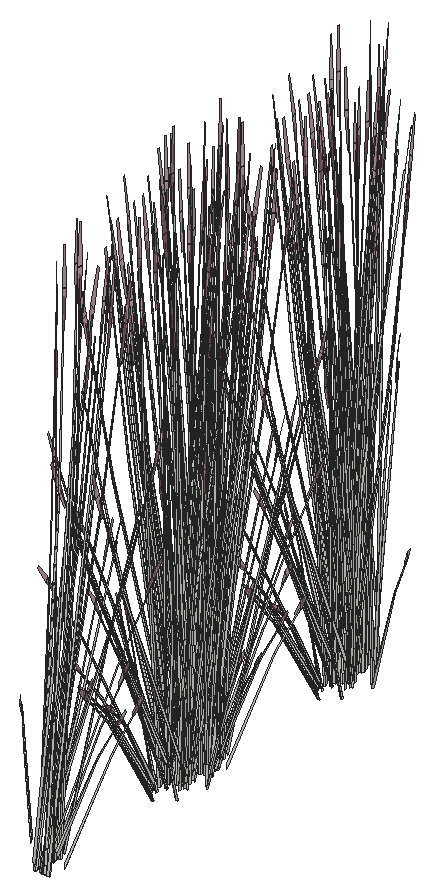
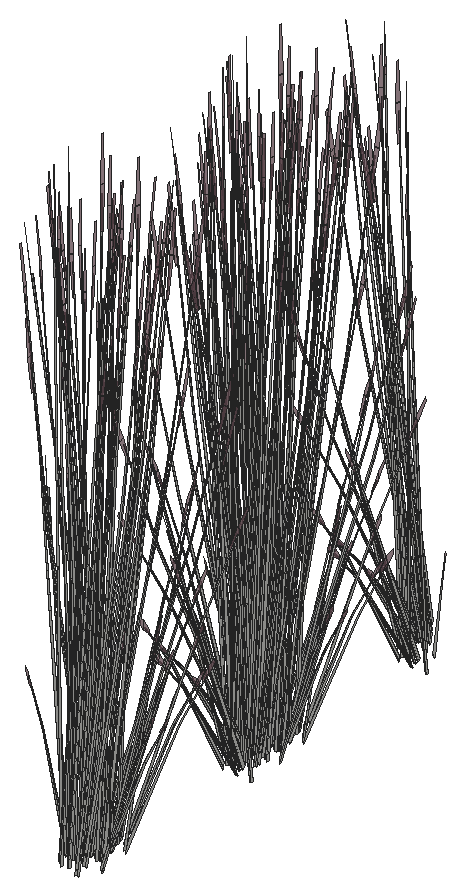
# SketchUp Ruby script. Lengths in inches.
U = 1.inch
M = Sketchup.active_model
def pt(a) = Geom::Point3d.new(a.map { |v| v * U })
def face(e, loops, mat)
  f = e.add_face(loops[0].map { |a| pt(a) })
  loops[1..].each { |l| e.add_face(l.map { |a| pt(a) }).erase! }
  f.material = f.back_material = mat if mat
  f
end
# faces: each face lists its corners as indices into pts; further lists are holes
def faces(e, pts, list, mat = nil) = list.each { |f| face(e, (f[0].is_a?(Array) ? f : [f]).map { |l| l.map { |i| pts[i] } }, mat) }
# xy, xz, yz: faces in a plane at the given z, y or x. An outline is a flat list of corners, or four numbers for a rectangle; further outlines are holes
def ring(l) = l.size == 4 ? [[l[0], l[1]], [l[2], l[1]], [l[2], l[3]], [l[0], l[3]]] : l.each_slice(2).to_a
def flat(e, list, mat, &to3) = list.each { |f| face(e, (f[0].is_a?(Array) ? f : [f]).map { |l| ring(l).map { |u, v| to3.(u, v) } }, mat) }
def xy(e, z, list, mat = nil) = flat(e, list, mat) { |x, y| [x, y, z] }
def xz(e, y, list, mat = nil) = flat(e, list, mat) { |x, z| [x, y, z] }
def yz(e, x, list, mat = nil) = flat(e, list, mat) { |y, z| [x, y, z] }
def lines(e, pts, list) = list.each { |a, b| e.add_line(pt(pts[a]), pt(pts[b])) }
# prism: a flat outline (further loops are holes) pulled along v
def prism(e, loops, v, mat = nil)
  f = face(e, loops, mat); d = Geom::Vector3d.new(v.map { |x| x * U })
  f.pushpull(f.normal.samedirection?(d) ? d.length : -d.length)
end
def box(e, o, s, mat = nil) = prism(e, [[o, [o[0] + s[0], o[1], o[2]], [o[0] + s[0], o[1] + s[1], o[2]], [o[0], o[1] + s[1], o[2]]]], [0, 0, s[2]], mat)
def at(x, y, z, deg = 0) = Geom::Transformation.translation(pt([x, y, z])) * Geom::Transformation.rotation(ORIGIN, Z_AXIS, deg.degrees)
def axes(o, x, y, z) = Geom::Transformation.new([*x, 0, *y, 0, *z, 0, *pt(o).to_a, 1])
def part(name) = M.definitions.add(name)
# library, detail: a bought-in or finely detailed component or shape, given as its bounding box
def library(name, o, s) = part(name).tap { |d| box(d.entities, o, s) }
def detail(e, o, s) = box(e.add_group.entities, o, s)
def put(e, d, t, mat = nil) = e.add_instance(d, t).tap { |i| i.material = mat if mat }
def group(e, t, mat = nil) = e.add_group.tap { |g| g.transformation = t; g.material = mat if mat }.entities
root = M.entities
M.materials.add("LightPink_Translucent").color = [144, 107, 117]
M.materials["LightPink_Translucent"].alpha = 0.75
c1 = part("blade")
p = [[2.15,0.21,22],[0,0.17,0],[0.09,0.45,0],[2.18,0.31,22],[2.29,0.31,22],[0.38,0.45,0],
  [2.48,0.24,33],[2.49,0.24,33],[2.48,0.22,33]]
faces(c1.entities,p,[[0,1,2,3],[4,5,2,3],[6,3,4,7],[8,0,3,6]])
c2 = part("seeds")
p = [[0.3,-0.1,1.38],[-0.01,-0.03,1.59],[-0.01,-0.03,0.03],[0.14,-0.07,-0.07],[0.29,-0.03,3],[0.15,0.01,3.11]]
faces(c2.entities,p,[[0,1,2,3],[1,0,4,5]],"LightPink_Translucent")
c3 = part("blade with seeds")
put(c3.entities,c1,at(0,0,0))
put(c3.entities,c2,axes([2.4,0.25,30.99],[1.5799,-0.05474,1.17369],[-0.12525,1.92788,0.29478],[-0.07173,-0.02425,1.56792]))
put(root,c3,axes([252.92,30.17,0.92],[0.32006,0,0],[0,0.68339,-0.37456],[0,0.15565,1.18819]))
put(root,c3,axes([252.79,30.52,0.79],[-0.3199,-0.00489,-0.03612],[0,-0.68339,0.36248],[-0.01005,0.15557,1.14929]))
put(root,c3,axes([252.1,29.93,1.13],[0.28825,0.29175,-0.21117],[-0.1388,0.61578,-0.36291],[0.00906,0.15119,1.15913]))
put(root,c3,axes([250.09,32.2,1.2],[0.10667,-0.27712,0.83364],[0.04209,0.43871,0.6125],[-0.07709,0.07855,0.18362]))
put(root,c3,axes([252.73,30.62,0.66],[-0.17867,0.3815,-0.22483],[-0.17867,-0.3815,0.22483],[0,0.12288,1.00865]))
put(root,c3,axes([251.96,30.66,1.13],[0.02983,0.6977,-0.21117],[-0.31064,0.04219,-0.36291],[-0.0547,0.09294,1.15913]))
put(root,c3,axes([252.07,30.39,0.8],[-0.12419,0.55096,-0.32471],[-0.25804,-0.26516,0.15627],[0,0.12701,1.04254]))
put(root,c3,axes([251.77,31.19,0.6875],[-0.1724,0.45959,-0.45255],[-0.21416,-0.41674,-0.11877],[-0.06908,0.11465,0.99892]))
put(root,c3,axes([252.08,31.97,0.88],[0.32044,0.19874,0.22322],[-0.08017,0.71038,-0.26485],[-0.05304,0.08891,1.19671]))
put(root,c3,axes([252.05,32.44,0.66],[-0.23955,0.30573,-0.36036],[-0.14318,-0.54821,0],[-0.05456,0.06963,1.14313]))
put(root,c3,axes([252.85,30.63,0.66],[0,0.61145,-0.36036],[-0.28637,0,0],[0,0.13926,1.14313]))
put(root,c3,axes([252.49,31.9,1.2],[-0.14411,-0.17581,0.83364],[0.18609,-0.17864,0.6125],[0.05019,0.15132,0.18362]))
put(root,c3,axes([252.27,32.35,0.91],[0.16003,0.61271,0],[-0.26773,0.34169,-0.37456],[-0.06098,0.07782,1.18819]))
put(root,c3,axes([252.53,32.56,0.28],[0.01865,-0.08828,1.27986],[0.23477,-0.25998,-0.19552],[0.07118,0.13456,0.218]))
put(root,c3,axes([252.13,29.92,1.26],[-0.00699,-0.5757,1.02533],[0.31645,0.14923,0.43413],[-0.07484,0.31502,0.96783]))
put(root,c3,axes([252.22,30.55,0.71],[0.09385,0.55983,-0.50233],[-0.27035,0.20162,-0.13184],[0.01037,0.18957,1.1088]))
put(root,c3,axes([250.37,32.48,0.28],[0.03433,0.06109,1.27986],[0.05822,0.56601,-0.19552],[-0.07609,0.1207,0.218]))
put(root,c3,axes([252.51,32.7,1.13],[-0.16414,-0.01918,0.76251],[0.10839,-0.40729,0.421],[0.06484,0.1447,0.59812]))
put(root,c3,axes([251.97,31.72,1.07],[0.00452,-0.20269,1.03788],[0.21585,-0.22641,-0.22321],[0.06663,0.2426,0.44375]))
put(root,c3,axes([250.99,33.41,1.2],[-0.00662,-0.36357,0.83364],[0.16552,0.25931,0.6125],[-0.03255,0.17329,0.18362]))
put(root,c3,axes([251.43,32.54,0.28],[0.04142,-0.03327,1.27986],[0.24917,0.18313,-0.19552],[0.00729,0.2064,0.218]))
put(root,c3,axes([250.86,32.62,1.24],[0.23252,-0.10828,0.04723],[0.05346,0.43623,-0.62638],[-0.01474,0.22082,0.56147]))
put(root,c3,axes([251.51,32.3,2.81],[0.12216,0.49718,-0.51563],[-0.25147,0.27708,0.06223],[0.02857,0.24022,0.72942]))
put(root,c3,axes([250.8,33.08,1.07],[0.08077,-0.09646,1.03788],[0.19942,0.29084,-0.22321],[-0.05936,0.25166,0.44375]))
put(root,c3,axes([252.15,43.34,1.07],[-0.07276,0.12376,1.03788],[-0.21789,-0.21662,-0.22321],[0.04039,-0.2694,0.44375]))
put(root,c3,axes([251.82,43.77,2.81],[-0.12216,-0.49718,-0.51563],[0.25147,-0.27708,0.06223],[-0.02857,-0.24022,0.72942]))
put(root,c3,axes([251.03,43.11,1.07],[-0.0155,0.20002,1.03788],[-0.22659,0.16744,-0.22321],[-0.05297,-0.25854,0.44375]))
put(root,c3,axes([251.61,42.67,0.28],[-0.04293,0.02203,1.27986],[-0.23742,-0.24798,-0.19552],[0.00398,-0.20684,0.218]))
put(root,c3,axes([252.33,44.26,2.81],[0.00666,-0.56559,-0.51563],[0.28045,0.03799,0.06223],[0.0296,-0.23961,0.72942]))
put(root,c3,axes([251.88,42.35,1.2],[0.03283,0.35655,0.83364],[-0.18215,-0.19748,0.6125],[0.0196,-0.18257,0.18362]))
put(root,c3,axes([250.95,42.78,1.2],[0.13352,0.21281,0.83364],[-0.19445,0.12793,0.6125],[-0.0416,-0.16355,0.18362]))
put(root,c3,axes([251.27,43.91,2.81],[-0.21825,-0.29555,-0.51563],[0.15511,-0.5179,0.06223],[-0.07907,-0.17646,0.72942]))
put(root,c3,axes([250.84,43.42,0.28],[-0.02479,0.08055,1.27986],[-0.25056,0.17367,-0.19552],[-0.06053,-0.15798,0.218]))
put(root,c3,axes([251.25,45.64,0.72],[-0.10512,-0.62701,-0.50685],[0.30279,-0.22582,-0.13303],[-0.01162,-0.21232,1.11879]))
put(root,c3,axes([252.66,43.72,0.28],[-0.03831,-0.04817,1.27986],[-0.0984,-0.53815,-0.19552],[0.06638,-0.14604,0.218]))
put(root,c3,axes([252.66,45.24,2.81],[0.1337,-0.48245,-0.51563],[0.23429,0.34287,0.06223],[0.07983,-0.1748,0.72942]))
put(root,c3,axes([251.21,43.84,0.91],[-0.16003,-0.61271,0],[0.26773,-0.34169,-0.37456],[0.06098,-0.07782,1.18819]))
put(root,c3,axes([251.56,43.1,0.74],[-0.17688,0.35078,-0.02825],[-0.16207,-0.38418,-0.1281],[-0.01141,-0.10886,0.42251]))
put(root,c3,axes([250.64,45.55,0.66],[0,-0.61145,-0.36036],[0.28637,0,0],[0,-0.13926,1.14313]))
put(root,c3,axes([251.43,43.74,0.66],[0.23955,-0.30573,-0.36036],[0.14318,0.54821,0],[0.05456,-0.06963,1.14313]))
put(root,c3,axes([252.85,44.8,1.07],[-0.09144,-0.01811,1.03788],[-0.09368,-0.48584,-0.22321],[0.11233,-0.13744,0.44375]))
put(root,c3,axes([251.71,44.99,0.6875],[0.1724,-0.45959,-0.45255],[0.21416,0.41674,-0.11877],[0.06908,-0.11465,0.99892]))
put(root,c3,axes([252.96,43.9,1.2],[-0.08525,0.31126,0.83364],[-0.07328,-0.41819,0.6125],[0.07041,-0.10479,0.18362]))
put(root,c3,axes([251.41,45.8,0.8],[0.12419,-0.55096,-0.32471],[0.25804,0.26516,0.15627],[0,-0.12701,1.04254]))
put(root,c3,axes([251.53,45.53,1.13],[-0.02983,-0.6977,-0.21117],[0.31064,-0.04219,-0.36291],[0.0547,-0.09294,1.15913]))
put(root,c3,axes([250.76,45.5625,0.66],[0.17867,-0.3815,-0.22483],[0.17867,0.3815,0.22483],[0,-0.12288,1.00865]))
put(root,c3,axes([250.6875,43.73,0.74],[-0.07384,0.49928,-0.02825],[-0.22725,-0.15358,-0.1281],[-0.0345,-0.08166,0.42251]))
put(root,c3,axes([251.38,46.26,1.13],[-0.28825,-0.29175,-0.21117],[0.1388,-0.61578,-0.36291],[-0.00906,-0.15119,1.15913]))
put(root,c3,axes([250.5625,46.01,0.91],[-0.32006,0,0],[0,-0.68339,-0.37456],[0,-0.15565,1.18819]))
put(root,c3,axes([250.62,44.79,1.07],[0.04997,0.17024,1.03788],[-0.11515,0.46273,-0.22321],[-0.11824,-0.1106,0.44375]))
put(root,c3,axes([251.49,43.98,0.66],[0.23879,0.15129,-0.22483],[-0.06012,0.53279,0.22483],[0.04814,-0.06144,1.00865]))
put(root,c3,axes([250.82,44.64,2.81],[-0.25586,-0.01472,-0.51563],[0.01718,-0.61995,0.06223],[-0.1084,-0.06542,0.72942]))
put(root,c3,axes([250.8125,45.83,0.88],[-0.23808,0.51407,0.22322],[-0.23822,-0.50866,-0.26485],[-0.00831,-0.14599,1.19671]))
put(root,c3,axes([251.57,46.07,0.96],[0.28839,0.29636,0.17466],[-0.1388,0.61578,0.36291],[0,-0.14195,1.16519]))
put(root,c3,axes([251.46,46.91,0.96],[0.06784,-0.72454,-0.17004],[0.32166,0.1263,0.37211],[-0.05621,-0.10006,1.13542]))
put(root,c3,axes([250.32,45.3,1.2],[0.16341,-0.04375,0.83364],[-0.10366,0.38551,0.6125],[-0.08075,-0.05783,0.18362]))
put(root,c3,axes([251.48,45.66,1.17],[-0.27795,0.03775,0.32471],[-0.02514,-0.62656,-0.15627],[0.04976,-0.0635,1.04254]))
put(root,c3,axes([250.76,46.12,0.99],[0,0.61145,0.36036],[-0.28637,0,0],[0,-0.13926,1.14313]))
put(root,c3,axes([252.39,43.99,0.92],[0.16003,-0.61271,0],[0.26773,0.34169,-0.37456],[0.06098,0.07782,1.18819]))
put(root,c3,axes([251.43,46.61,0.8],[-0.15376,-0.51322,-0.32471],[0.2329,-0.3614,0.15627],[-0.04976,-0.0635,1.04254]))
put(root,c3,axes([251.47,45.89,0.91],[0.11128,0.68373,0.33208],[-0.31797,0.23776,0.13031],[0.00389,-0.12563,1.15295]))
put(root,c3,axes([253.02,46.41,0.63],[-0.16485,0.07338,1.02759],[-0.02624,-0.58408,0.05882],[0.11546,-0.08841,0.58473]))
put(root,c3,axes([253.32,45.89,0.83],[-0.15869,-0.39099,-0.04709],[0.1738,-0.35825,-0.21349],[0.04925,-0.02522,0.70419]))
put(root,c3,axes([251.41,46.43,1.17],[-0.12419,0.55096,0.32471],[-0.25804,-0.26516,-0.15627],[0,-0.12701,1.04254]))
put(root,c3,axes([251.87,45.94,0.79],[0,-0.70749,0],[0.32006,0,0],[0,0,1.30246]))
put(root,c3,axes([252.25,44.31,0.99],[-0.23955,-0.30573,0.36036],[0.14318,-0.54821,0],[0.05456,0.06963,1.14313]))
put(root,c3,axes([252.72,46.46,2.81],[0.22491,-0.27005,-0.51563],[0.12534,0.55588,0.06223],[0.10867,-0.06315,0.72942]))
put(root,c3,axes([251.3,46.81,0.6875],[-0.26625,-0.10025,-0.45255],[0.05619,-0.61836,-0.11877],[-0.07946,-0.07493,0.99892]))
put(root,c3,axes([251.71,45.5,0.91],[-0.21222,0.5549,0.33208],[-0.25213,-0.48983,0.13031],[0.05116,-0.05538,1.15295]))
put(root,c3,axes([251.95,46.49,0.86],[-0.23808,-0.52628,-0.0445],[0.23822,-0.5266,0],[-0.00831,-0.01838,1.27426]))
put(root,c3,axes([251.35,44.59,0.99],[-0.07394,0.60768,0.12804],[-0.27057,-0.17197,0.25465],[0.04674,-0.00296,1.1642]))
put(root,c3,axes([251.23,45.08,0.35],[-0.25194,0.2448,0.93574],[-0.08019,-0.7024,0.36359],[0.1547,0.01169,1.0643]))
put(root,c3,axes([251.91,45.26,1.09],[0.04938,-0.54569,0.10509],[0.24125,0.09472,-0.30009],[0.0439,0.05603,0.91989]))
put(root,c3,axes([251.49,46.56,0.91],[0.32351,0.12883,0.33208],[-0.06584,0.72759,0.13031],[-0.04728,-0.07026,1.15295]))
put(root,c3,axes([253.2,46.03,0.28],[-0.01338,-0.09283,1.27986],[0.09278,-0.54301,-0.19552],[0.09359,-0.00781,0.218]))
put(root,c3,axes([250.44,45.93,0.28],[0.00649,0.09636,1.27986],[-0.13086,0.50324,-0.19552],[-0.09295,-0.02537,0.218]))
put(root,c3,axes([251.81,45.4,1.17],[-0.15376,-0.51322,0.32471],[0.2329,-0.3614,-0.15627],[0.04976,0.0635,1.04254]))
put(root,c3,axes([251.01,47.75,0.66],[-0.06012,-0.53279,-0.22483],[0.23879,-0.15129,0.22483],[-0.04814,-0.06144,1.00865]))
put(root,c3,axes([251.32,47.72,0.99],[0.27504,-0.16229,0.12804],[0.06792,0.60396,0.25465],[-0.02453,-0.088,1.1642]))
put(root,c3,axes([251.89,45.4375,1.13],[0.25843,-0.40595,-0.21117],[0.17185,0.5736,-0.36291],[0.06376,0.05825,1.15913]))
put(root,c3,axes([250.95,47.98,0.66],[-0.23955,-0.30573,-0.36036],[0.14318,-0.54821,0],[-0.05456,-0.06963,1.14313]))
put(root,c3,axes([252.54,44.36,0.66],[0.23955,0.30573,-0.36036],[-0.14318,0.54821,0],[0.05456,0.06963,1.14313]))
put(root,c3,axes([252.08,46.1,0.79],[0.28637,0,0],[0,0.63302,0],[0,0,1.29484]))
put(root,c3,axes([251.6,46.9,1.13],[-0.25843,0.40595,-0.21117],[-0.17185,-0.5736,-0.36291],[-0.06376,-0.05825,1.15913]))
put(root,c3,axes([252.16,44.62,0.99],[-0.27504,0.16229,0.12804],[-0.06792,-0.60396,0.25465],[0.02453,0.088,1.1642]))
put(root,c3,axes([252.47,44.59,0.66],[0.06012,0.53279,-0.22483],[-0.23879,0.15129,0.22483],[0.04814,0.06144,1.00865]))
put(root,c3,axes([251.99,45.78,0.92],[-0.32351,-0.12883,0.35707],[0.06584,-0.72759,0.14012],[0.04728,0.07026,1.23973]))
put(root,c3,axes([251.73,47.58,0.79],[-0.08351,-0.52716,0],[0.23848,-0.18461,0],[0,0,1.1204]))
put(root,c3,axes([251.57,47.08,1.09],[-0.04938,0.54569,0.10509],[-0.24125,-0.09472,-0.30009],[-0.0439,-0.05603,0.91989]))
put(root,c3,axes([252.05,47.5,0.78],[0.26872,-0.20746,-0.13933],[0.09442,0.59762,0.00006],[0.02966,-0.02293,1.26212]))
put(root,c3,axes([252.14,47.75,0.99],[0.07394,-0.60768,0.12804],[0.27057,0.17197,0.25465],[-0.04674,0.00296,1.1642]))
put(root,c3,axes([252.08,46.375,0.8],[0.17867,0.39495,0],[-0.17867,0.39495,0],[0,0,1.22851]))
put(root,c3,axes([252.5625,46.2,0.99],[-0.2011,-0.44539,0.12804],[0.20266,-0.432,0.25465],[-0.02221,0.09096,1.1642]))
put(root,c3,axes([252.1875,45.53,0.6875],[0.26625,0.10025,-0.45255],[-0.05619,0.61836,-0.11877],[0.07946,0.07493,0.99892]))
put(root,c3,axes([253.36,46.61,1.2],[-0.15814,0.10094,0.83364],[0.07444,-0.41719,0.6125],[0.0839,0.02855,0.18362]))
put(root,c3,axes([251.67,47.82,0.79],[-0.25804,-0.27452,0],[0.12419,-0.5704,0],[0,0,1.1809]))
put(root,c3,axes([251.89,47.08,0.98],[-0.24993,-0.49214,-0.18284],[0.21031,-0.55263,0.40012],[-0.0673,0.05757,1.22088]))
put(root,c3,axes([251.23,48.03,0.99],[0.23955,0.30573,0.36036],[-0.14318,0.54821,0],[-0.05456,-0.06963,1.14313]))
put(root,c3,axes([252.07,45.91,1.17],[0.12419,-0.55096,0.32471],[0.25804,0.26516,-0.15627],[0,0.12701,1.04254]))
put(root,c3,axes([252.03,46.23,0.86],[0,0.70714,-0.04091],[-0.32006,0,0],[0,0.02222,1.30182]))
put(root,c3,axes([252.05,45.73,0.8],[0.15376,0.51322,-0.32471],[-0.2329,0.3614,0.15627],[0.04976,0.0635,1.04254]))
put(root,c3,axes([251.09,48.35,0.91],[-0.16003,0.61271,0],[-0.26773,-0.34169,-0.37456],[-0.06098,-0.07782,1.18819]))
put(root,c3,axes([252.73,46.22,0.99],[0,-0.61145,0.36036],[0.28637,0,0],[0,0.13926,1.14313]))
put(root,c3,axes([252.01,46.68,1.17],[0.27795,-0.03775,0.32471],[0.02514,0.62656,-0.15627],[-0.04976,0.0635,1.04254]))
put(root,c3,axes([252.18,46.04,1.09],[0.23848,-0.17832,0.10509],[0.08351,0.5092,-0.30009],[0,0.11207,0.91989]))
put(root,c3,axes([251.76,46.98,0.8],[-0.27795,0.03775,-0.32471],[-0.02514,-0.62656,0.15627],[-0.04976,0.0635,1.04254]))
put(root,c3,axes([253.07,47.28,1.07],[-0.06164,-0.15038,1.03788],[0.0802,-0.49748,-0.22321],[0.12472,0.06739,0.44375]))
put(root,c3,axes([251.97,47.83,0.79],[0.25804,0.27452,0],[-0.12419,0.5704,0],[0,0,1.26978]))
put(root,c3,axes([252.07,48.43,0.78],[-0.15803,-0.61485,-0.03732],[0.26773,-0.34169,0.37456],[-0.06597,0.05854,1.1876]))
put(root,c3,axes([252.01,46.95,1.09],[0.1891,0.36737,0.10509],[-0.15773,0.41447,-0.30009],[-0.0439,0.05603,0.91989]))
put(root,c3,axes([252.5,47.58,2.81],[0.25586,0.01472,-0.51563],[-0.01718,0.61995,0.06223],[0.1084,0.06542,0.72942]))
put(root,c3,axes([252.21,48.08,0.99],[0.23955,-0.30573,0.36036],[0.14318,0.54821,0],[-0.05456,0.06963,1.14313]))
put(root,c3,axes([251.875,47.6,0.86],[0.11128,0.70245,-0.04364],[-0.31797,0.24614,0],[0.00389,0.02453,1.2496]))
put(root,c3,axes([252,48.36,0.66],[-0.23879,-0.15129,-0.22483],[0.06012,-0.53279,0.22483],[-0.04814,0.06144,1.00865]))
put(root,c3,axes([250.27,47.27,1.07],[0.08895,0.05019,1.03788],[0.05733,0.5127,-0.22321],[-0.12083,0.09597,0.44375]))
put(root,c3,axes([252.92,46.32,0.92],[0.32006,0,0],[0,0.68339,-0.37456],[0,0.15565,1.18819]))
put(root,c3,axes([252.79,46.67,0.79],[-0.3199,-0.00489,-0.03612],[0,-0.68339,0.36248],[-0.01005,0.15557,1.14929]))
put(root,c3,axes([252.1,46.08,1.13],[0.28825,0.29175,-0.21117],[-0.1388,0.61578,-0.36291],[0.00906,0.15119,1.15913]))
put(root,c3,axes([250.09,48.35,1.2],[0.10667,-0.27712,0.83364],[0.04209,0.43871,0.6125],[-0.07709,0.07855,0.18362]))
put(root,c3,axes([252.73,46.77,0.66],[-0.17867,0.3815,-0.22483],[-0.17867,-0.3815,0.22483],[0,0.12288,1.00865]))
put(root,c3,axes([251.96,46.81,1.13],[0.02983,0.6977,-0.21117],[-0.31064,0.04219,-0.36291],[-0.0547,0.09294,1.15913]))
put(root,c3,axes([252.07,46.54,0.8],[-0.12419,0.55096,-0.32471],[-0.25804,-0.26516,0.15627],[0,0.12701,1.04254]))
put(root,c3,axes([251.77,47.34,0.6875],[-0.1724,0.45959,-0.45255],[-0.21416,-0.41674,-0.11877],[-0.06908,0.11465,0.99892]))
put(root,c3,axes([252.08,48.12,0.88],[0.32044,0.19874,0.22322],[-0.08017,0.71038,-0.26485],[-0.05304,0.08891,1.19671]))
put(root,c3,axes([252.05,48.6,0.66],[-0.23955,0.30573,-0.36036],[-0.14318,-0.54821,0],[-0.05456,0.06963,1.14313]))
put(root,c3,axes([252.85,46.79,0.66],[0,0.61145,-0.36036],[-0.28637,0,0],[0,0.13926,1.14313]))
put(root,c3,axes([252.49,48.06,1.2],[-0.14411,-0.17581,0.83364],[0.18609,-0.17864,0.6125],[0.05019,0.15132,0.18362]))
put(root,c3,axes([252.27,48.5,0.91],[0.16003,0.61271,0],[-0.26773,0.34169,-0.37456],[-0.06098,0.07782,1.18819]))
put(root,c3,axes([252.53,48.71,0.28],[0.01865,-0.08828,1.27986],[0.23477,-0.25998,-0.19552],[0.07118,0.13456,0.218]))
put(root,c3,axes([252.13,46.08,1.26],[-0.00699,-0.5757,1.02533],[0.31645,0.14923,0.43413],[-0.07484,0.31502,0.96783]))
put(root,c3,axes([252.22,46.7,0.71],[0.09385,0.55983,-0.50233],[-0.27035,0.20162,-0.13184],[0.01037,0.18957,1.1088]))
put(root,c3,axes([250.37,48.63,0.28],[0.03433,0.06109,1.27986],[0.05822,0.56601,-0.19552],[-0.07609,0.1207,0.218]))
put(root,c3,axes([252.51,48.86,1.13],[-0.16414,-0.01918,0.76251],[0.10839,-0.40729,0.421],[0.06484,0.1447,0.59812]))
put(root,c3,axes([251.97,47.87,1.07],[0.00452,-0.20269,1.03788],[0.21585,-0.22641,-0.22321],[0.06663,0.2426,0.44375]))
put(root,c3,axes([250.99,49.56,1.2],[-0.00662,-0.36357,0.83364],[0.16552,0.25931,0.6125],[-0.03255,0.17329,0.18362]))
put(root,c3,axes([251.43,48.6875,0.28],[0.04142,-0.03327,1.27986],[0.24917,0.18313,-0.19552],[0.00729,0.2064,0.218]))
put(root,c3,axes([250.86,48.77,1.24],[0.23252,-0.10828,0.04723],[0.05346,0.43623,-0.62638],[-0.01474,0.22082,0.56147]))
put(root,c3,axes([251.51,48.45,2.81],[0.12216,0.49718,-0.51563],[-0.25147,0.27708,0.06223],[0.02857,0.24022,0.72942]))
put(root,c3,axes([250.8,49.24,1.07],[0.08077,-0.09646,1.03788],[0.19942,0.29084,-0.22321],[-0.05936,0.25166,0.44375]))
put(root,c3,axes([252.15,59.79,1.07],[-0.07276,0.12376,1.03788],[-0.21789,-0.21662,-0.22321],[0.04039,-0.2694,0.44375]))
put(root,c3,axes([251.82,60.22,2.81],[-0.12216,-0.49718,-0.51563],[0.25147,-0.27708,0.06223],[-0.02857,-0.24022,0.72942]))
put(root,c3,axes([251.03,59.56,1.07],[-0.0155,0.20002,1.03788],[-0.22659,0.16744,-0.22321],[-0.05297,-0.25854,0.44375]))
put(root,c3,axes([251.61,59.12,0.28],[-0.04293,0.02203,1.27986],[-0.23742,-0.24798,-0.19552],[0.00398,-0.20684,0.218]))
put(root,c3,axes([252.33,60.71,2.81],[0.00666,-0.56559,-0.51563],[0.28045,0.03799,0.06223],[0.0296,-0.23961,0.72942]))
put(root,c3,axes([251.88,58.81,1.2],[0.03283,0.35655,0.83364],[-0.18215,-0.19748,0.6125],[0.0196,-0.18257,0.18362]))
put(root,c3,axes([250.95,59.23,1.2],[0.13352,0.21281,0.83364],[-0.19445,0.12793,0.6125],[-0.0416,-0.16355,0.18362]))
put(root,c3,axes([251.27,60.36,2.81],[-0.21825,-0.29555,-0.51563],[0.15511,-0.5179,0.06223],[-0.07907,-0.17646,0.72942]))
put(root,c3,axes([250.84,59.875,0.28],[-0.02479,0.08055,1.27986],[-0.25056,0.17367,-0.19552],[-0.06053,-0.15798,0.218]))
put(root,c3,axes([251.25,62.09,0.72],[-0.10512,-0.62701,-0.50685],[0.30279,-0.22582,-0.13303],[-0.01162,-0.21232,1.11879]))
put(root,c3,axes([252.66,60.17,0.28],[-0.03831,-0.04817,1.27986],[-0.0984,-0.53815,-0.19552],[0.06638,-0.14604,0.218]))
put(root,c3,axes([252.66,61.69,2.81],[0.1337,-0.48245,-0.51563],[0.23429,0.34287,0.06223],[0.07983,-0.1748,0.72942]))
put(root,c3,axes([251.21,60.29,0.91],[-0.16003,-0.61271,0],[0.26773,-0.34169,-0.37456],[0.06098,-0.07782,1.18819]))
put(root,c3,axes([251.56,59.55,0.74],[-0.17688,0.35078,-0.02825],[-0.16207,-0.38418,-0.1281],[-0.01141,-0.10886,0.42251]))
put(root,c3,axes([250.64,62,0.66],[0,-0.61145,-0.36036],[0.28637,0,0],[0,-0.13926,1.14313]))
put(root,c3,axes([251.43,60.19,0.66],[0.23955,-0.30573,-0.36036],[0.14318,0.54821,0],[0.05456,-0.06963,1.14313]))
put(root,c3,axes([252.85,61.25,1.07],[-0.09144,-0.01811,1.03788],[-0.09368,-0.48584,-0.22321],[0.11233,-0.13744,0.44375]))
put(root,c3,axes([251.71,61.45,0.6875],[0.1724,-0.45959,-0.45255],[0.21416,0.41674,-0.11877],[0.06908,-0.11465,0.99892]))
put(root,c3,axes([252.96,60.35,1.2],[-0.08525,0.31126,0.83364],[-0.07328,-0.41819,0.6125],[0.07041,-0.10479,0.18362]))
put(root,c3,axes([251.41,62.25,0.8],[0.12419,-0.55096,-0.32471],[0.25804,0.26516,0.15627],[0,-0.12701,1.04254]))
put(root,c3,axes([251.53,61.98,1.13],[-0.02983,-0.6977,-0.21117],[0.31064,-0.04219,-0.36291],[0.0547,-0.09294,1.15913]))
put(root,c3,axes([250.76,62.01,0.66],[0.17867,-0.3815,-0.22483],[0.17867,0.3815,0.22483],[0,-0.12288,1.00865]))
put(root,c3,axes([250.6875,60.1875,0.74],[-0.07384,0.49928,-0.02825],[-0.22725,-0.15358,-0.1281],[-0.0345,-0.08166,0.42251]))
put(root,c3,axes([251.38,62.71,1.13],[-0.28825,-0.29175,-0.21117],[0.1388,-0.61578,-0.36291],[-0.00906,-0.15119,1.15913]))
put(root,c3,axes([250.5625,62.47,0.91],[-0.32006,0,0],[0,-0.68339,-0.37456],[0,-0.15565,1.18819]))
put(root,c3,axes([250.62,61.24,1.07],[0.04997,0.17024,1.03788],[-0.11515,0.46273,-0.22321],[-0.11824,-0.1106,0.44375]))
put(root,c3,axes([251.49,60.43,0.66],[0.23879,0.15129,-0.22483],[-0.06012,0.53279,0.22483],[0.04814,-0.06144,1.00865]))
put(root,c3,axes([250.82,61.09,2.81],[-0.25586,-0.01472,-0.51563],[0.01718,-0.61995,0.06223],[-0.1084,-0.06542,0.72942]))
put(root,c3,axes([250.8125,62.28,0.88],[-0.23808,0.51407,0.22322],[-0.23822,-0.50866,-0.26485],[-0.00831,-0.14599,1.19671]))
put(root,c3,axes([251.57,62.52,0.96],[0.28839,0.29636,0.17466],[-0.1388,0.61578,0.36291],[0,-0.14195,1.16519]))
put(root,c3,axes([251.46,63.36,0.96],[0.06784,-0.72454,-0.17004],[0.32166,0.1263,0.37211],[-0.05621,-0.10006,1.13542]))
put(root,c3,axes([250.32,61.76,1.2],[0.16341,-0.04375,0.83364],[-0.10366,0.38551,0.6125],[-0.08075,-0.05783,0.18362]))
put(root,c3,axes([251.48,62.11,1.17],[-0.27795,0.03775,0.32471],[-0.02514,-0.62656,-0.15627],[0.04976,-0.0635,1.04254]))
put(root,c3,axes([250.76,62.57,0.99],[0,0.61145,0.36036],[-0.28637,0,0],[0,-0.13926,1.14313]))
put(root,c3,axes([252.39,60.44,0.92],[0.16003,-0.61271,0],[0.26773,0.34169,-0.37456],[0.06098,0.07782,1.18819]))
put(root,c3,axes([251.43,63.0625,0.8],[-0.15376,-0.51322,-0.32471],[0.2329,-0.3614,0.15627],[-0.04976,-0.0635,1.04254]))
put(root,c3,axes([251.47,62.34,0.91],[0.11128,0.68373,0.33208],[-0.31797,0.23776,0.13031],[0.00389,-0.12563,1.15295]))
put(root,c3,axes([253.02,62.86,0.63],[-0.16485,0.07338,1.02759],[-0.02624,-0.58408,0.05882],[0.11546,-0.08841,0.58473]))
put(root,c3,axes([253.32,62.34,0.83],[-0.15869,-0.39099,-0.04709],[0.1738,-0.35825,-0.21349],[0.04925,-0.02522,0.70419]))
put(root,c3,axes([251.41,62.875,1.17],[-0.12419,0.55096,0.32471],[-0.25804,-0.26516,-0.15627],[0,-0.12701,1.04254]))
put(root,c3,axes([251.87,62.4,0.79],[0,-0.70749,0],[0.32006,0,0],[0,0,1.30246]))
put(root,c3,axes([252.25,60.76,0.99],[-0.23955,-0.30573,0.36036],[0.14318,-0.54821,0],[0.05456,0.06963,1.14313]))
put(root,c3,axes([252.72,62.91,2.81],[0.22491,-0.27005,-0.51563],[0.12534,0.55588,0.06223],[0.10867,-0.06315,0.72942]))
put(root,c3,axes([251.3,63.26,0.6875],[-0.26625,-0.10025,-0.45255],[0.05619,-0.61836,-0.11877],[-0.07946,-0.07493,0.99892]))
put(root,c3,axes([251.71,61.95,0.91],[-0.21222,0.5549,0.33208],[-0.25213,-0.48983,0.13031],[0.05116,-0.05538,1.15295]))
put(root,c3,axes([251.95,62.94,0.86],[-0.23808,-0.52628,-0.0445],[0.23822,-0.5266,0],[-0.00831,-0.01838,1.27426]))
put(root,c3,axes([251.35,61.04,0.99],[-0.07394,0.60768,0.12804],[-0.27057,-0.17197,0.25465],[0.04674,-0.00296,1.1642]))
put(root,c3,axes([251.23,61.53,0.35],[-0.25194,0.2448,0.93574],[-0.08019,-0.7024,0.36359],[0.1547,0.01169,1.0643]))
put(root,c3,axes([251.91,61.71,1.09],[0.04938,-0.54569,0.10509],[0.24125,0.09472,-0.30009],[0.0439,0.05603,0.91989]))
put(root,c3,axes([251.49,63.01,0.91],[0.32351,0.12883,0.33208],[-0.06584,0.72759,0.13031],[-0.04728,-0.07026,1.15295]))
put(root,c3,axes([253.2,62.48,0.28],[-0.01338,-0.09283,1.27986],[0.09278,-0.54301,-0.19552],[0.09359,-0.00781,0.218]))
put(root,c3,axes([250.44,62.39,0.28],[0.00649,0.09636,1.27986],[-0.13086,0.50324,-0.19552],[-0.09295,-0.02537,0.218]))
put(root,c3,axes([251.81,61.86,1.17],[-0.15376,-0.51322,0.32471],[0.2329,-0.3614,-0.15627],[0.04976,0.0635,1.04254]))
put(root,c3,axes([251.01,64.2,0.66],[-0.06012,-0.53279,-0.22483],[0.23879,-0.15129,0.22483],[-0.04814,-0.06144,1.00865]))
put(root,c3,axes([251.32,64.17,0.99],[0.27504,-0.16229,0.12804],[0.06792,0.60396,0.25465],[-0.02453,-0.088,1.1642]))
put(root,c3,axes([251.89,61.89,1.13],[0.25843,-0.40595,-0.21117],[0.17185,0.5736,-0.36291],[0.06376,0.05825,1.15913]))
put(root,c3,axes([250.95,64.43,0.66],[-0.23955,-0.30573,-0.36036],[0.14318,-0.54821,0],[-0.05456,-0.06963,1.14313]))
put(root,c3,axes([252.54,60.81,0.66],[0.23955,0.30573,-0.36036],[-0.14318,0.54821,0],[0.05456,0.06963,1.14313]))
put(root,c3,axes([252.08,62.55,0.79],[0.28637,0,0],[0,0.63302,0],[0,0,1.29484]))
put(root,c3,axes([251.6,63.35,1.13],[-0.25843,0.40595,-0.21117],[-0.17185,-0.5736,-0.36291],[-0.06376,-0.05825,1.15913]))
put(root,c3,axes([252.16,61.07,0.99],[-0.27504,0.16229,0.12804],[-0.06792,-0.60396,0.25465],[0.02453,0.088,1.1642]))
put(root,c3,axes([252.47,61.04,0.66],[0.06012,0.53279,-0.22483],[-0.23879,0.15129,0.22483],[0.04814,0.06144,1.00865]))
put(root,c3,axes([251.99,62.23,0.92],[-0.32351,-0.12883,0.35707],[0.06584,-0.72759,0.14012],[0.04728,0.07026,1.23973]))
put(root,c3,axes([251.73,64.03,0.79],[-0.08351,-0.52716,0],[0.23848,-0.18461,0],[0,0,1.1204]))
put(root,c3,axes([251.57,63.53,1.09],[-0.04938,0.54569,0.10509],[-0.24125,-0.09472,-0.30009],[-0.0439,-0.05603,0.91989]))
put(root,c3,axes([252.05,63.95,0.78],[0.26872,-0.20746,-0.13933],[0.09442,0.59762,0.00006],[0.02966,-0.02293,1.26212]))
put(root,c3,axes([252.14,64.2,0.99],[0.07394,-0.60768,0.12804],[0.27057,0.17197,0.25465],[-0.04674,0.00296,1.1642]))
put(root,c3,axes([252.08,62.83,0.8],[0.17867,0.39495,0],[-0.17867,0.39495,0],[0,0,1.22851]))
